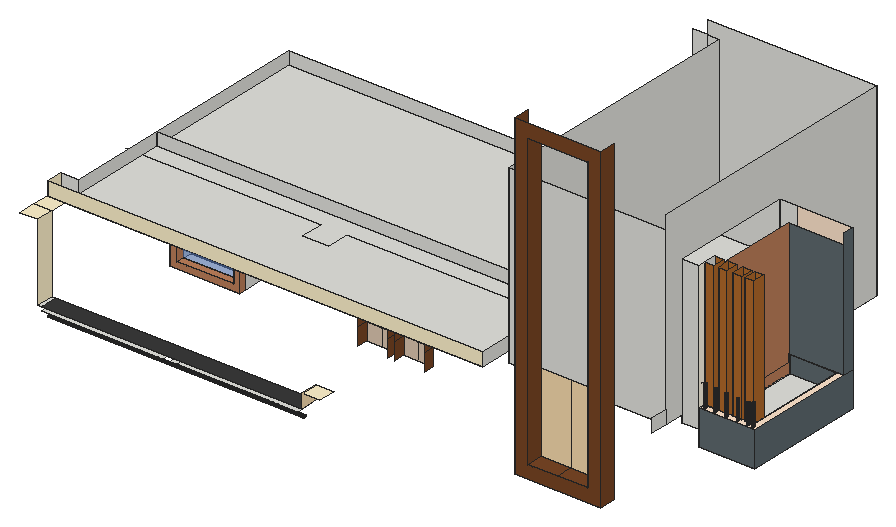
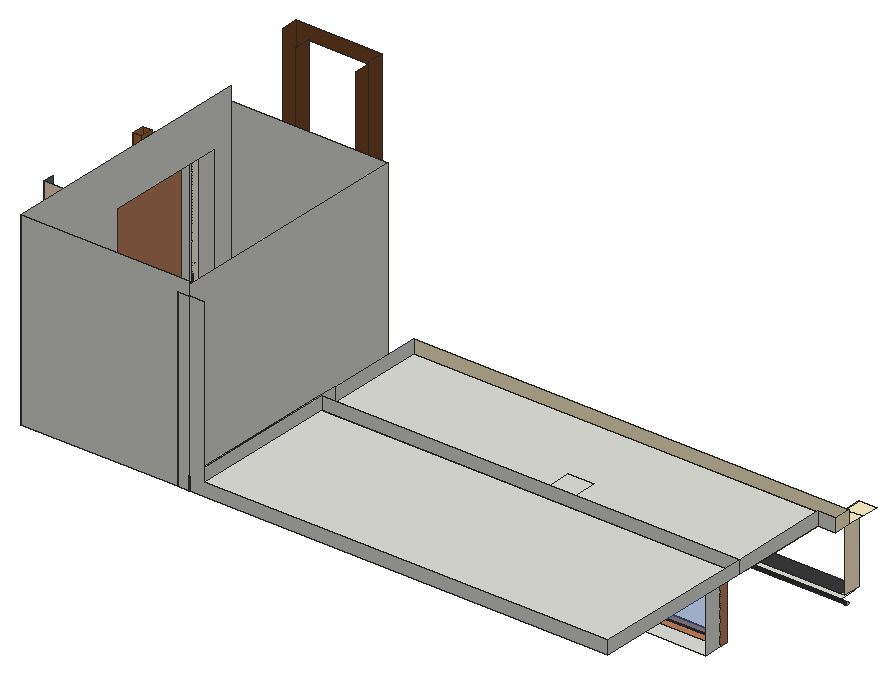
# SketchUp Ruby script. Lengths in inches.
U = 1.inch
M = Sketchup.active_model
def pt(a) = Geom::Point3d.new(a.map { |v| v * U })
def face(e, loops, mat)
  f = e.add_face(loops[0].map { |a| pt(a) })
  loops[1..].each { |l| e.add_face(l.map { |a| pt(a) }).erase! }
  f.material = f.back_material = mat if mat
  f
end
# faces: each face lists its corners as indices into pts; further lists are holes
def faces(e, pts, list, mat = nil) = list.each { |f| face(e, (f[0].is_a?(Array) ? f : [f]).map { |l| l.map { |i| pts[i] } }, mat) }
# xy, xz, yz: faces in a plane at the given z, y or x. An outline is a flat list of corners, or four numbers for a rectangle; further outlines are holes
def ring(l) = l.size == 4 ? [[l[0], l[1]], [l[2], l[1]], [l[2], l[3]], [l[0], l[3]]] : l.each_slice(2).to_a
def flat(e, list, mat, &to3) = list.each { |f| face(e, (f[0].is_a?(Array) ? f : [f]).map { |l| ring(l).map { |u, v| to3.(u, v) } }, mat) }
def xy(e, z, list, mat = nil) = flat(e, list, mat) { |x, y| [x, y, z] }
def xz(e, y, list, mat = nil) = flat(e, list, mat) { |x, z| [x, y, z] }
def yz(e, x, list, mat = nil) = flat(e, list, mat) { |y, z| [x, y, z] }
def lines(e, pts, list) = list.each { |a, b| e.add_line(pt(pts[a]), pt(pts[b])) }
# prism: a flat outline (further loops are holes) pulled along v
def prism(e, loops, v, mat = nil)
  f = face(e, loops, mat); d = Geom::Vector3d.new(v.map { |x| x * U })
  f.pushpull(f.normal.samedirection?(d) ? d.length : -d.length)
end
def box(e, o, s, mat = nil) = prism(e, [[o, [o[0] + s[0], o[1], o[2]], [o[0] + s[0], o[1] + s[1], o[2]], [o[0], o[1] + s[1], o[2]]]], [0, 0, s[2]], mat)
def at(x, y, z, deg = 0) = Geom::Transformation.translation(pt([x, y, z])) * Geom::Transformation.rotation(ORIGIN, Z_AXIS, deg.degrees)
def axes(o, x, y, z) = Geom::Transformation.new([*x, 0, *y, 0, *z, 0, *pt(o).to_a, 1])
def part(name) = M.definitions.add(name)
# library, detail: a bought-in or finely detailed component or shape, given as its bounding box
def library(name, o, s) = part(name).tap { |d| box(d.entities, o, s) }
def detail(e, o, s) = box(e.add_group.entities, o, s)
def put(e, d, t, mat = nil) = e.add_instance(d, t).tap { |i| i.material = mat if mat }
def group(e, t, mat = nil) = e.add_group.tap { |g| g.transformation = t; g.material = mat if mat }.entities
root = M.entities
M.materials.add("[Color C01]").color = [221, 199, 177]
M.materials.add("[Color C01]1").color = [255, 229, 204]
M.materials.add("[Color D01]").color = [255, 242, 204]
M.materials.add("[Color M07]").color = [58, 58, 58]
M.materials.add("[Formica Beige]1").color = [247, 219, 174]
M.materials.add("[Formica Beige]2").color = [249, 221, 176]
M.materials.add("[Formica Graystone]1").color = [255, 249, 231]
M.materials.add("[Formica Laminate Dark]").color = [50, 53, 60]
M.materials.add("[Formica Speckled Grey]").color = [94, 105, 111]
M.materials.add("[Translucent Glass Blue]").color = [100, 149, 237]
M.materials["[Translucent Glass Blue]"].alpha = 0.5
M.materials.add("[Wood Bamboo]").color = [177, 105, 43]
M.materials.add("[Wood Veneer 01]").color = [120, 70, 37]
M.materials.add("[Wood Veneer 02]").color = [190, 128, 91]
xy(root,267,[[139.94,388.54,331.76,436.38]])
xy(root,267,[[139.94,366.98,331.76,388.54]],"[Wood Veneer 02]")
xy(root,276.5625,[[58.17,25.9375,392.86,73.63],[411.53,25.9375,430.19,73.63],[430.19,25.9375,763.2,73.63]])
xy(root,284.55,[[157.5,366.98,314.2,388.54]],"[Wood Veneer 02]")
xy(root,288.4375,[[47.7,25.9375,58.17,73.63]])
xy(root,288.4375,[[58.17,25.9375,775.53,73.63]],"[Color M07]")
xy(root,298.625,[[1322.15,73.86,1559.21,119.17]],"[Wood Veneer 01]")
xy(root,326.25,[[775.53,25.9375,824.4,73.63]],"[Color D01]")
xy(root,334.49,[[1358.02,73.86,1440.68,119.17],[1440.68,73.86,1523.35,119.17]],"[Wood Veneer 01]")
xy(root,405.79,[[662.82,359.29,704.31,388.54],[704.31,359.29,745.81,388.54],[764.54,359.29,805.45,388.54],[805.45,359.29,846.36,388.54]],"[Wood Veneer 01]")
xy(root,420.08,[[648.52,388.54,860.65,436.38]])
xy(root,420.08,[[648.52,359.29,860.65,388.54]],"[Wood Veneer 01]")
xy(root,423.9375,[[958.75,388.54,1164.68,436.38]])
xy(root,425.51,[[157.5,366.98,314.2,388.54]],"[Wood Veneer 02]")
xy(root,438.77,[[1713.03,219.81,1866.15,557.62]],"[Formica Speckled Grey]")
xy(root,443.06,[[139.94,388.54,331.76,436.38]])
xy(root,443.06,[[139.94,366.98,331.76,388.54]],"[Wood Veneer 02]")
xy(root,481.82,[[1665.33,219.81,1713.03,557.62],[1713.03,240.49,1736.96,274.61],[1736.96,240.49,1750.4,240.49,1750.4,274.61,1774.34,274.61,1774.34,240.49,1790.96,240.49,1790.96,274.61,1814.9,274.61,1814.9,240.49,1823.34,240.49,1823.34,274.61,1847.28,274.61,1847.28,533.61,1713.03,533.61,1713.03,274.61,1736.96,274.61],[1750.4,240.49,1774.34,274.61],[1790.96,240.49,1814.9,274.61],
  [1823.34,240.49,1847.28,274.61]])
xy(root,500.125,[[0,119.17,47.7,166.1],[47.7,119.17,47.7,388.54,539.84,388.54,539.84,324.79,609.42,324.79,609.42,388.54,1198.27,388.54,1198.27,119.17],[1232.71,166.04,1665.33,388.54],[539.84,324.79,609.42,324.79,609.42,388.54,1201.41,388.54,1201.41,436.38,47.7,436.38,47.7,388.54,539.84,388.54],[1201.41,388.54,1665.33,436.38],
  [47.7,436.38,1198.27,890.39],[1198.27,436.38,1201.41,436.38,1198.27,890.39],[1201.41,436.38,1201.41,890.39,1198.27,890.39],[1201.41,436.38,1232.71,890.39],[1232.71,436.38,1665.33,890.39]])
xy(root,500.125,[[0,25.9375,47.7,73.63],[0,73.63,47.7,119.17]],"[Color D01]")
xy(root,501.875,[[1232.71,388.54,1665.33,436.38]])
xy(root,533.38,[[1722.85,227.29,1722.08,227.4,1721.35,227.69,1720.73,228.17,1720.25,228.79,1719.96,229.52,1719.85,230.29,1719.96,231.07,1720.25,231.79,1720.73,232.41,1721.35,232.89,1722.08,233.19,1722.85,233.29,1723.63,233.19,1724.35,232.89,1724.97,232.41,1725.45,231.79,1725.75,231.07,1725.85,230.29,1725.75,229.52,1725.45,228.79,1724.97,228.17,1724.35,227.69,1723.63,227.4],[1750.54,227.29,1749.76,227.4,1749.04,227.69,1748.42,228.17,1747.94,228.79,1747.64,229.52,1747.54,230.29,1747.64,231.07,1747.94,231.79,1748.42,232.41,1749.04,232.89,1749.76,233.19,1750.54,233.29,1751.32,233.19,1752.04,232.89,1752.66,232.41,1753.14,231.79,1753.4375,231.07,1753.54,230.29,1753.4375,229.52,1753.14,228.79,1752.66,228.17,1752.04,227.69,1751.32,227.4],[1780.92,227.29,1780.14,227.4,1779.42,227.69,1778.79,228.17,1778.32,228.79,1778.02,229.52,1777.92,230.29,1778.02,231.07,1778.32,231.79,1778.79,232.41,1779.42,232.89,1780.14,233.19,1780.92,233.29,1781.69,233.19,1782.42,232.89,1783.04,232.41,1783.51,231.79,1783.8125,231.07,1783.92,230.29,1783.8125,229.52,1783.51,228.79,1783.04,228.17,1782.42,227.69,1781.69,227.4],[1811.85,227.29,1811.08,227.4,1810.35,227.69,1809.73,228.17,1809.25,228.79,1808.96,229.52,1808.85,230.29,1808.96,231.07,1809.25,231.79,1809.73,232.41,1810.35,232.89,1811.08,233.19,1811.85,233.29,1812.63,233.19,1813.35,232.89,1813.97,232.41,1814.45,231.79,1814.75,231.07,1814.85,230.29,1814.75,229.52,1814.45,228.79,1813.97,228.17,1813.35,227.69,1812.63,227.4],[1840.85,227.29,1840.08,227.4,1839.35,227.69,1838.73,228.17,1838.25,228.79,1837.96,229.52,1837.85,230.29,1837.96,231.07,1838.25,231.79,1838.73,232.41,1839.35,232.89,1840.08,233.19,1840.85,233.29,1841.63,233.19,1842.35,232.89,1842.97,232.41,1843.45,231.79,1843.75,231.07,1843.85,230.29,1843.75,229.52,1843.45,228.79,1842.97,228.17,1842.35,227.69,1841.63,227.4],
  [1855.17,227.29,1854.39,227.4,1853.67,227.69,1853.04,228.17,1852.57,228.79,1852.27,229.52,1852.17,230.29,1852.27,231.07,1852.57,231.79,1853.04,232.41,1853.67,232.89,1854.39,233.19,1855.17,233.29,1855.94,233.19,1856.67,232.89,1857.29,232.41,1857.76,231.79,1858.0625,231.07,1858.17,230.29,1858.0625,229.52,1857.76,228.79,1857.29,228.17,1856.67,227.69,1855.94,227.4],[1713.03,528.45,1847.28,533.61],[1847.28,528.45,1866.15,533.61],[1713.03,533.61,1866.15,556.25],[1713.03,556.25,1866.15,557.62]])
xy(root,533.38,[[[1713.03,219.81,1866.15,219.81,1866.15,528.45,1847.28,528.45,1847.28,240.49,1713.03,240.49],[1780.92,227.29,1780.14,227.4,1779.42,227.69,1778.79,228.17,1778.32,228.79,1778.02,229.52,1777.92,230.29,1778.02,231.07,1778.32,231.79,1778.79,232.41,1779.42,232.89,1780.14,233.19,1780.92,233.29,1781.69,233.19,1782.42,232.89,1783.04,232.41,1783.51,231.79,1783.8125,231.07,1783.92,230.29,1783.8125,229.52,1783.51,228.79,1783.04,228.17,1782.42,227.69,1781.69,227.4],[1811.85,227.29,1811.08,227.4,1810.35,227.69,1809.73,228.17,1809.25,228.79,1808.96,229.52,1808.85,230.29,1808.96,231.07,1809.25,231.79,1809.73,232.41,1810.35,232.89,1811.08,233.19,1811.85,233.29,1812.63,233.19,1813.35,232.89,1813.97,232.41,1814.45,231.79,1814.75,231.07,1814.85,230.29,1814.75,229.52,1814.45,228.79,1813.97,228.17,1813.35,227.69,1812.63,227.4],[1750.54,227.29,1749.76,227.4,1749.04,227.69,1748.42,228.17,1747.94,228.79,1747.64,229.52,1747.54,230.29,1747.64,231.07,1747.94,231.79,1748.42,232.41,1749.04,232.89,1749.76,233.19,1750.54,233.29,1751.32,233.19,1752.04,232.89,1752.66,232.41,1753.14,231.79,1753.4375,231.07,1753.54,230.29,1753.4375,229.52,1753.14,228.79,1752.66,228.17,1752.04,227.69,1751.32,227.4],[1840.85,227.29,1840.08,227.4,1839.35,227.69,1838.73,228.17,1838.25,228.79,1837.96,229.52,1837.85,230.29,1837.96,231.07,1838.25,231.79,1838.73,232.41,1839.35,232.89,1840.08,233.19,1840.85,233.29,1841.63,233.19,1842.35,232.89,1842.97,232.41,1843.45,231.79,1843.75,231.07,1843.85,230.29,1843.75,229.52,1843.45,228.79,1842.97,228.17,1842.35,227.69,1841.63,227.4],[1855.17,227.29,1854.39,227.4,1853.67,227.69,1853.04,228.17,1852.57,228.79,1852.27,229.52,1852.17,230.29,1852.27,231.07,1852.57,231.79,1853.04,232.41,1853.67,232.89,1854.39,233.19,1855.17,233.29,1855.94,233.19,1856.67,232.89,1857.29,232.41,1857.76,231.79,1858.0625,231.07,1858.17,230.29,1858.0625,229.52,1857.76,228.79,1857.29,228.17,1856.67,227.69,1855.94,227.4],[1722.85,227.29,1722.08,227.4,1721.35,227.69,1720.73,228.17,1720.25,228.79,1719.96,229.52,1719.85,230.29,1719.96,231.07,1720.25,231.79,1720.73,232.41,1721.35,232.89,1722.08,233.19,1722.85,233.29,1723.63,233.19,1724.35,232.89,1724.97,232.41,1725.45,231.79,1725.75,231.07,1725.85,230.29,1725.75,229.52,1725.45,228.79,1724.97,228.17,1724.35,227.69,1723.63,227.4]]],"[Color C01]1")
xz(root,73.86,[[[1322.15,298.625,1559.21,1175.6875],[1358.02,334.49,1523.35,1139.82]]],"[Wood Veneer 01]")
xz(root,119.17,[[0,500.125,1198.27,536.125]],"[Color D01]")
xz(root,119.17,[[1358.02,334.49,1440.68,552.78],[1440.68,334.49,1523.35,552.78]],"[Formica Beige]1")
xz(root,166.04,[[1232.71,500.125,1665.33,980.3125]])
xz(root,166.1,[[0,500.125,47.7,536.125]])
xz(root,219.81,[[1665.33,481.82,1713.03,885.01]])
xz(root,219.81,[[1713.03,438.77,1866.15,533.38]],"[Formica Speckled Grey]")
xz(root,240.49,[[1713.03,481.82,1736.96,533.38],[1736.96,481.82,1750.4,533.38],[1750.4,481.82,1774.34,533.38],[1774.34,481.82,1790.96,533.38],[1790.96,481.82,1814.9,533.38],
  [1814.9,481.82,1823.34,533.38],[1823.34,481.82,1847.28,533.38]])
xz(root,240.49,[[1713.03,533.38,1736.96,885.01],[1750.4,533.38,1774.34,885.01],[1790.96,533.38,1814.9,885.01],[1823.34,533.38,1847.28,885.01]],"[Wood Bamboo]")
xz(root,274.61,[[1713.03,481.82,1736.96,885.01],[1750.4,481.82,1774.34,885.01],[1790.96,481.82,1814.9,885.01],[1823.34,481.82,1847.28,885.01]],"[Wood Bamboo]")
xz(root,366.98,[[[139.94,267,331.76,443.06],[157.5,284.55,314.2,425.51]]],"[Wood Veneer 02]")
xz(root,388.54,[[1198.27,500.125,1201.41,536.125],[1232.71,500.125,1433.37,501.875],[1433.37,500.125,1457.06,501.875],[1457.06,500.125,1665.33,501.875]])
xz(root,388.54,[[662.82,256.87,704.31,303.93],[704.31,256.87,745.81,303.93],[764.54,256.87,805.45,303.93],[805.45,256.87,846.36,303.93],[662.82,303.93,704.31,348.4375],
  [704.31,303.93,745.81,348.4375],[764.54,303.93,805.45,348.4375],[805.45,303.93,846.36,348.4375],[662.82,348.4375,704.31,405.79],[704.31,348.4375,745.81,405.79],
  [764.54,348.4375,805.45,405.79],[805.45,348.4375,846.36,405.79]],"[Color C01]")
xz(root,388.54,[[157.5,284.55,314.2,425.51]],"[Translucent Glass Blue]")
xz(root,436.38,[[47.7,500.125,1198.27,536.125],[1198.27,500.125,1201.41,536.125],[1232.71,500.125,1665.33,501.875]])
xz(root,528.45,[[1713.03,533.38,1866.15,855.83]],"[Formica Speckled Grey]")
xz(root,533.61,[[1713.03,481.82,1847.28,533.38]],"[Formica Speckled Grey]")
xz(root,557.62,[[1665.33,481.82,1713.03,885.01]])
xz(root,557.62,[[1713.03,533.38,1866.15,885.01]],"[Color C01]1")
xz(root,557.62,[[1713.03,438.77,1866.15,533.38]],"[Formica Speckled Grey]")
xz(root,890.39,[[47.7,500.125,1198.27,500.125,1198.27,980.9375,1159.05,980.9375,1159.05,536.125,47.7,536.125],[1198.27,500.125,1201.41,536.125],[1201.41,500.125,1201.41,536.125,1201.79,536.125,1201.79,980.3125,1232.71,980.3125,1232.71,500.125],[1232.71,500.125,1665.33,500.125,1665.33,1016.9375,1201.79,1016.9375,1201.79,980.3125,1232.71,980.3125]])
yz(root,0,[[119.17,500.125,166.1,536.125]],"[Color D01]")
yz(root,47.7,[[166.1,500.125,436.38,536.125],[436.38,500.125,890.39,536.125]])
yz(root,47.7,[[25.9375,288.4375,73.63,500.125]],"[Color D01]")
yz(root,58.17,[[51.27,251.25,50.49,251.35,49.77,251.65,49.15,252.13,48.67,252.75,48.37,253.48,48.27,254.25,48.37,255.03,48.67,255.75,49.15,256.375,49.77,256.85,50.49,257.15,51.27,257.25,52.04,257.15,52.77,256.85,53.39,256.375,53.87,255.75,54.17,255.03,54.27,254.25,54.17,253.48,53.87,252.75,53.39,252.13,52.77,251.65,52.04,251.35]])
yz(root,139.94,[[388.54,267,436.38,443.06]])
yz(root,139.94,[[366.98,267,388.54,443.06]],"[Wood Veneer 02]")
yz(root,157.5,[[366.98,284.55,388.54,425.51]],"[Wood Veneer 02]")
yz(root,314.2,[[366.98,284.55,388.54,425.51]],"[Wood Veneer 02]")
yz(root,331.76,[[388.54,267,436.38,443.06]])
yz(root,331.76,[[366.98,267,388.54,443.06]],"[Wood Veneer 02]")
yz(root,662.82,[[359.29,256.87,388.54,303.93],[359.29,303.93,388.54,348.4375],[359.29,348.4375,388.54,405.79]],"[Wood Veneer 01]")
yz(root,745.81,[[359.29,256.87,388.54,303.93],[359.29,303.93,388.54,348.4375],[359.29,348.4375,388.54,405.79]],"[Wood Veneer 01]")
yz(root,764.54,[[359.29,256.87,388.54,303.93],[359.29,303.93,388.54,348.4375],[359.29,348.4375,388.54,405.79]],"[Wood Veneer 01]")
yz(root,775.53,[[25.9375,288.4375,73.63,326.25]],"[Formica Beige]2")
yz(root,846.36,[[359.29,256.87,388.54,303.93],[359.29,303.93,388.54,348.4375],[359.29,348.4375,388.54,405.79]],"[Wood Veneer 01]")
yz(root,1198.27,[[119.17,500.125,388.54,536.125],[436.38,500.125,890.39,536.125]])
yz(root,1201.41,[[388.54,500.125,436.38,536.125],[436.38,500.125,890.39,536.125]])
yz(root,1232.71,[[166.04,500.125,388.54,500.125,388.54,501.875,890.39,501.875,890.39,980.3125,166.04,980.3125],[436.38,500.125,890.39,501.875]])
yz(root,1322.15,[[73.86,298.625,119.17,1175.6875]],"[Wood Veneer 01]")
yz(root,1358.02,[[73.86,334.49,119.17,1139.82]],"[Wood Veneer 01]")
yz(root,1523.35,[[73.86,334.49,119.17,1139.82]],"[Wood Veneer 01]")
yz(root,1559.21,[[73.86,298.625,119.17,1175.6875]],"[Wood Veneer 01]")
yz(root,1665.33,[[219.81,481.82,388.54,500.125],[388.54,481.82,436.38,500.125],[436.38,481.82,557.62,500.125],[119.17,500.125,166.04,536.125],[166.04,500.125,166.04,1016.9375,890.39,1016.9375,890.39,500.125,557.62,500.125,557.62,885.01,219.81,885.01,219.81,500.125],
  [388.54,500.125,436.38,501.875]])
yz(root,1713.03,[[219.81,438.77,557.62,481.82],[219.81,481.82,240.49,533.38],[240.49,481.82,240.49,885.01,274.61,885.01,274.61,855.83,248.98,855.83,248.98,510.99,274.61,510.99,274.61,481.82],[533.61,481.82,556.25,533.38],[556.25,481.82,557.62,533.38],
  [248.98,510.99,274.61,855.83]])
yz(root,1713.03,[[[219.81,533.38,240.49,885.01],[229.09,588.26,228.18,588.375,227.34,588.73,226.61,589.28,226.06,590.01,225.71,590.85,225.59,591.76,225.71,592.66,226.06,593.51,226.61,594.23,227.34,594.79,228.18,595.14,229.09,595.26,229.99,595.14,230.84,594.79,231.5625,594.23,232.12,593.51,232.47,592.66,232.59,591.76,232.47,590.85,232.12,590.01,231.5625,589.28,230.84,588.73,229.99,588.375]]],"[Formica Graystone]1")
yz(root,1713.03,[[274.61,481.82,533.61,481.82,533.61,533.38,528.45,533.38,528.45,510.99,274.61,510.99],[274.61,510.99,528.45,855.83]],"[Wood Veneer 02]")
yz(root,1736.96,[[240.49,481.82,274.61,885.01]],"[Wood Bamboo]")
yz(root,1750.4,[[240.49,481.82,274.61,885.01]],"[Wood Bamboo]")
yz(root,1774.34,[[240.49,481.82,274.61,885.01]],"[Wood Bamboo]")
yz(root,1790.96,[[240.49,481.82,274.61,885.01]],"[Wood Bamboo]")
yz(root,1814.9,[[240.49,481.82,274.61,885.01]],"[Wood Bamboo]")
yz(root,1823.34,[[240.49,481.82,274.61,885.01]],"[Wood Bamboo]")
yz(root,1847.28,[[240.49,481.82,274.61,533.38],[274.61,481.82,533.61,533.38]])
yz(root,1847.28,[[240.49,533.38,274.61,885.01]],"[Wood Bamboo]")
yz(root,1866.15,[[219.81,438.77,557.62,533.38],[528.45,533.38,557.62,885.01]],"[Formica Speckled Grey]")
p = [[58.17,50.49,251.35],[58.17,51.27,251.25],[763.2,51.27,251.25],[763.2,50.49,251.35],[58.17,52.04,251.35],[763.2,52.04,251.35],
  [58.17,49.77,251.65],[763.2,49.77,251.65],[58.17,52.77,251.65],[763.2,52.77,251.65],[58.17,49.15,252.13],[763.2,49.15,252.13],
  [58.17,53.39,252.13],[763.2,53.39,252.13],[58.17,48.67,252.75],[763.2,48.67,252.75],[58.17,53.87,252.75],[763.2,53.87,252.75],
  [58.17,48.37,253.48],[763.2,48.37,253.48],[58.17,54.17,253.48],[763.2,54.17,253.48],[58.17,48.27,254.25],[763.2,48.27,254.25],
  [58.17,54.27,254.25],[763.2,54.27,254.25],[58.17,48.37,255.03],[763.2,48.37,255.03],[58.17,54.17,255.03],[763.2,54.17,255.03],
  [58.17,48.67,255.75],[763.2,48.67,255.75],[58.17,53.87,255.75],[763.2,53.87,255.75],[58.17,49.15,256.375],[763.2,49.15,256.375],
  [58.17,53.39,256.375],[763.2,53.39,256.375],[58.17,49.77,256.85],[763.2,49.77,256.85],[58.17,52.77,256.85],[763.2,52.77,256.85],
  [58.17,50.49,257.15],[763.2,50.49,257.15],[58.17,52.04,257.15],[763.2,52.04,257.15],[58.17,51.27,257.25],[763.2,51.27,257.25],
  [1201.41,436.38,500.125],[1198.27,890.39,500.125],[1198.27,890.39,536.125],[1201.41,436.38,536.125],[1722.08,227.4,533.38],[1722.85,227.29,533.38],
  [1722.85,227.29,593.51],[1722.08,227.4,593.51],[1723.63,227.4,533.38],[1723.63,227.4,593.51],[1749.76,227.4,533.38],[1750.54,227.29,533.38],
  [1750.54,227.29,591.76],[1749.76,227.4,591.76],[1751.32,227.4,533.38],[1751.32,227.4,591.76],[1780.14,227.4,533.38],[1780.92,227.29,533.38],
  [1780.92,227.29,589.07],[1780.14,227.4,589.07],[1781.69,227.4,533.38],[1781.69,227.4,589.07],[1811.08,227.4,533.38],[1811.85,227.29,533.38],
  [1811.85,227.29,588.32],[1811.08,227.4,588.32],[1812.63,227.4,533.38],[1812.63,227.4,588.32],[1840.08,227.4,533.38],[1840.85,227.29,533.38],
  [1840.85,227.29,588.82],[1840.08,227.4,588.82],[1841.63,227.4,533.38],[1841.63,227.4,588.82],[1854.39,227.4,533.38],[1855.17,227.29,533.38],
  [1855.17,227.29,592.19],[1854.39,227.4,592.19],[1855.94,227.4,533.38],[1855.94,227.4,592.19],[1721.35,227.69,533.38],[1721.35,227.69,593.51],
  [1724.35,227.69,533.38],[1724.35,227.69,593.51],[1749.04,227.69,533.38],[1749.04,227.69,591.76],[1752.04,227.69,533.38],[1752.04,227.69,591.76],
  [1779.42,227.69,533.38],[1779.42,227.69,589.07],[1782.42,227.69,533.38],[1782.42,227.69,589.07],[1810.35,227.69,533.38],[1810.35,227.69,588.32],
  [1813.35,227.69,533.38],[1813.35,227.69,588.32],[1839.35,227.69,533.38],[1839.35,227.69,588.82],[1842.35,227.69,533.38],[1842.35,227.69,588.82],
  [1853.67,227.69,533.38],[1853.67,227.69,592.19],[1856.67,227.69,533.38],[1856.67,227.69,592.19],[1720.73,228.17,533.38],[1720.73,228.17,593.51],
  [1724.97,228.17,533.38],[1724.97,228.17,593.51],[1748.42,228.17,533.38],[1748.42,228.17,591.76],[1752.66,228.17,533.38],[1752.66,228.17,591.76],
  [1778.79,228.17,533.38],[1778.79,228.17,589.07],[1783.04,228.17,533.38],[1783.04,228.17,589.07],[1809.73,228.17,533.38],[1809.73,228.17,588.32],
  [1813.97,228.17,533.38],[1813.97,228.17,588.32],[1838.73,228.17,533.38],[1838.73,228.17,588.82],[1842.97,228.17,533.38],[1842.97,228.17,588.82],
  [1853.04,228.17,533.38],[1853.04,228.17,592.19],[1857.29,228.17,533.38],[1857.29,228.17,592.19],[1720.25,228.79,533.38],[1720.25,228.79,593.51],
  [1725.45,228.79,533.38],[1725.45,228.79,593.51],[1747.94,228.79,533.38],[1747.94,228.79,591.76],[1753.14,228.79,533.38],[1753.14,228.79,591.76],
  [1778.32,228.79,533.38],[1778.32,228.79,589.07],[1783.51,228.79,533.38],[1783.51,228.79,589.07],[1809.25,228.79,533.38],[1809.25,228.79,588.32],
  [1814.45,228.79,533.38],[1814.45,228.79,588.32],[1838.25,228.79,533.38],[1838.25,228.79,588.82],[1843.45,228.79,533.38],[1843.45,228.79,588.82],
  [1852.57,228.79,533.38],[1852.57,228.79,592.19],[1857.76,228.79,533.38],[1857.76,228.79,592.19],[1719.96,229.52,533.38],[1719.96,229.52,593.51],
  [1725.75,229.52,533.38],[1725.75,229.52,593.51],[1747.64,229.52,533.38],[1747.64,229.52,591.76],[1753.4375,229.52,533.38],[1753.4375,229.52,591.76],
  [1778.02,229.52,533.38],[1778.02,229.52,589.07],[1783.8125,229.52,533.38],[1783.8125,229.52,589.07],[1808.96,229.52,533.38],[1808.96,229.52,588.32],
  [1814.75,229.52,533.38],[1814.75,229.52,588.32],[1837.96,229.52,533.38],[1837.96,229.52,588.82],[1843.75,229.52,533.38],[1843.75,229.52,588.82],
  [1852.27,229.52,533.38],[1852.27,229.52,592.19],[1858.0625,229.52,533.38],[1858.0625,229.52,592.19],[1719.85,230.29,533.38],[1719.85,230.29,593.51],
  [1725.85,230.29,533.38],[1725.85,230.29,593.51],[1747.54,230.29,533.38],[1747.54,230.29,591.76],[1753.54,230.29,533.38],[1753.54,230.29,591.76],
  [1777.92,230.29,533.38],[1777.92,230.29,589.07],[1783.92,230.29,533.38],[1783.92,230.29,589.07],[1808.85,230.29,533.38],[1808.85,230.29,588.32],
  [1814.85,230.29,533.38],[1814.85,230.29,588.32],[1837.85,230.29,533.38],[1837.85,230.29,588.82],[1843.85,230.29,533.38],[1843.85,230.29,588.82],
  [1852.17,230.29,533.38],[1852.17,230.29,592.19],[1858.17,230.29,533.38],[1858.17,230.29,592.19],[1719.96,231.07,533.38],[1719.96,231.07,593.51],
  [1725.75,231.07,533.38],[1725.75,231.07,593.51],[1747.64,231.07,533.38],[1747.64,231.07,591.76],[1753.4375,231.07,533.38],[1753.4375,231.07,591.76],
  [1778.02,231.07,533.38],[1778.02,231.07,589.07],[1783.8125,231.07,533.38],[1783.8125,231.07,589.07],[1808.96,231.07,533.38],[1808.96,231.07,588.32],
  [1814.75,231.07,533.38],[1814.75,231.07,588.32],[1837.96,231.07,533.38],[1837.96,231.07,588.82],[1843.75,231.07,533.38],[1843.75,231.07,588.82],
  [1852.27,231.07,533.38],[1852.27,231.07,592.19],[1858.0625,231.07,533.38],[1858.0625,231.07,592.19],[1720.25,231.79,533.38],[1720.25,231.79,593.51],
  [1725.45,231.79,533.38],[1725.45,231.79,593.51],[1747.94,231.79,533.38],[1747.94,231.79,591.76],[1753.14,231.79,533.38],[1753.14,231.79,591.76],
  [1778.32,231.79,533.38],[1778.32,231.79,589.07],[1783.51,231.79,533.38],[1783.51,231.79,589.07],[1809.25,231.79,533.38],[1809.25,231.79,588.32],
  [1814.45,231.79,533.38],[1814.45,231.79,588.32],[1838.25,231.79,533.38],[1838.25,231.79,588.82],[1843.45,231.79,533.38],[1843.45,231.79,588.82],
  [1852.57,231.79,533.38],[1852.57,231.79,592.19],[1857.76,231.79,533.38],[1857.76,231.79,592.19],[1720.73,232.41,533.38],[1720.5,232.12,593.51],
  [1720.73,232.41,593.51],[1724.97,232.41,533.38],[1724.97,232.41,593.51],[1725.2,232.12,593.51],[1748.42,232.41,533.38],[1748.42,232.41,591.76],
  [1752.66,232.41,533.38],[1752.66,232.41,591.76],[1778.79,232.41,533.38],[1778.79,232.41,589.07],[1783.04,232.41,533.38],[1783.04,232.41,589.07],
  [1809.73,232.41,533.38],[1809.73,232.41,588.32],[1813.97,232.41,533.38],[1813.97,232.41,588.32],[1838.73,232.41,533.38],[1838.73,232.41,588.82],
  [1842.97,232.41,533.38],[1842.97,232.41,588.82],[1853.04,232.41,533.38],[1853.04,232.41,592.19],[1857.29,232.41,533.38],[1857.29,232.41,592.19],
  [1721.35,232.89,533.38],[1721.35,232.89,593.51],[1724.35,232.89,533.38],[1724.35,232.89,593.51],[1749.04,232.89,533.38],[1748.65,232.59,591.76],
  [1749.04,232.89,591.76],[1752.04,232.89,533.38],[1752.04,232.89,591.76],[1752.44,232.59,591.76],[1779.42,232.89,533.38],[1779.42,232.89,589.07],
  [1782.42,232.89,533.38],[1782.42,232.89,589.07],[1810.35,232.89,533.38],[1810.35,232.89,588.32],[1813.35,232.89,533.38],[1813.35,232.89,588.32],
  [1839.35,232.89,533.38],[1839.35,232.89,588.82],[1842.35,232.89,533.38],[1842.35,232.89,588.82],[1853.67,232.89,533.38],[1853.67,232.89,592.19],
  [1856.67,232.89,533.38],[1856.67,232.89,592.19],[1722.08,233.19,533.38],[1722.08,233.19,593.51],[1723.63,233.19,533.38],[1723.63,233.19,593.51],
  [1749.76,233.19,533.38],[1749.76,233.19,591.76],[1751.32,233.19,533.38],[1751.32,233.19,591.76],[1780.14,233.19,533.38],[1780.14,233.19,589.07],
  [1781.69,233.19,533.38],[1781.69,233.19,589.07],[1811.08,233.19,533.38],[1811.08,233.19,588.32],[1812.63,233.19,533.38],[1812.63,233.19,588.32],
  [1840.08,233.19,533.38],[1840.08,233.19,588.82],[1841.63,233.19,533.38],[1841.63,233.19,588.82],[1854.39,233.19,533.38],[1854.39,233.19,592.19],
  [1855.94,233.19,533.38],[1855.94,233.19,592.19],[1722.85,233.29,533.38],[1722.85,233.29,593.51],[1750.54,233.29,533.38],[1750.54,233.29,591.76],
  [1780.92,233.29,533.38],[1780.92,233.29,589.07],[1811.85,233.29,533.38],[1811.85,233.29,588.32],[1840.85,233.29,533.38],[1840.85,233.29,588.82],
  [1855.17,233.29,533.38],[1855.17,233.29,592.19],[0,388.54,500.125],[47.7,388.54,500.125]]
faces(root,p,[[0,1,2,3],[1,4,5,2],[6,0,3,7],[4,8,9,5],[10,6,7,11],[8,12,13,9],[14,10,11,15],[12,16,17,13],
  [18,14,15,19],[16,20,21,17],[22,18,19,23],[20,24,25,21],[26,22,23,27],[24,28,29,25],[30,26,27,31],[28,32,33,29],
  [34,30,31,35],[32,36,37,33],[38,34,35,39],[36,40,41,37],[42,38,39,43],[40,44,45,41],[46,42,43,47],[44,46,47,45],
  [52,53,54,55],[53,56,57,54],[58,59,60,61],[59,62,63,60],[64,65,66,67],[65,68,69,66],[70,71,72,73],[71,74,75,72],
  [76,77,78,79],[77,80,81,78],[82,83,84,85],[83,86,87,84],[88,52,55,89],[56,90,91,57],[92,58,61,93],[62,94,95,63],
  [96,64,67,97],[68,98,99,69],[100,70,73,101],[74,102,103,75],[104,76,79,105],[80,106,107,81],[108,82,85,109],[86,110,111,87],
  [112,88,89,113],[90,114,115,91],[116,92,93,117],[94,118,119,95],[120,96,97,121],[98,122,123,99],[124,100,101,125],[102,126,127,103],
  [128,104,105,129],[106,130,131,107],[132,108,109,133],[110,134,135,111],[136,112,113,137],[114,138,139,115],[140,116,117,141],[118,142,143,119],
  [144,120,121,145],[122,146,147,123],[148,124,125,149],[126,150,151,127],[152,128,129,153],[130,154,155,131],[156,132,133,157],[134,158,159,135],
  [160,136,137,161],[138,162,163,139],[164,140,141,165],[142,166,167,143],[168,144,145,169],[146,170,171,147],[172,148,149,173],[150,174,175,151],
  [176,152,153,177],[154,178,179,155],[180,156,157,181],[158,182,183,159],[184,160,161,185],[162,186,187,163],[188,164,165,189],[166,190,191,167],
  [192,168,169,193],[170,194,195,171],[196,172,173,197],[174,198,199,175],[200,176,177,201],[178,202,203,179],[204,180,181,205],[182,206,207,183],
  [208,184,185,209],[186,210,211,187],[212,188,189,213],[190,214,215,191],[216,192,193,217],[194,218,219,195],[220,196,197,221],[198,222,223,199],
  [224,200,201,225],[202,226,227,203],[228,204,205,229],[206,230,231,207],[232,208,209,233],[210,234,235,211],[236,212,213,237],[214,238,239,215],
  [240,216,217,241],[218,242,243,219],[244,220,221,245],[222,246,247,223],[248,224,225,249],[226,250,251,227],[252,228,229,253],[230,254,255,231],
  [256,232,233,257,258],[234,259,260,261,235],[262,236,237,263],[238,264,265,239],[266,240,241,267],[242,268,269,243],[270,244,245,271],[246,272,273,247],
  [274,248,249,275],[250,276,277,251],[278,252,253,279],[254,280,281,255],[282,256,258,283],[259,284,285,260],[286,262,263,287,288],[264,289,290,291,265],
  [292,266,267,293],[268,294,295,269],[296,270,271,297],[272,298,299,273],[300,274,275,301],[276,302,303,277],[304,278,279,305],[280,306,307,281],
  [308,282,283,309],[284,310,311,285],[312,286,288,313],[289,314,315,290],[316,292,293,317],[294,318,319,295],[320,296,297,321],[298,322,323,299],
  [324,300,301,325],[302,326,327,303],[328,304,305,329],[306,330,331,307],[332,308,309,333],[310,332,333,311],[334,312,313,335],[314,334,335,315],
  [336,316,317,337],[318,336,337,319],[338,320,321,339],[322,338,339,323],[340,324,325,341],[326,340,341,327],[342,328,329,343],[330,342,343,331]],"[Formica Laminate Dark]")
faces(root,p,[[48,49,50,51]])
lines(root,p,[[344,345]])
